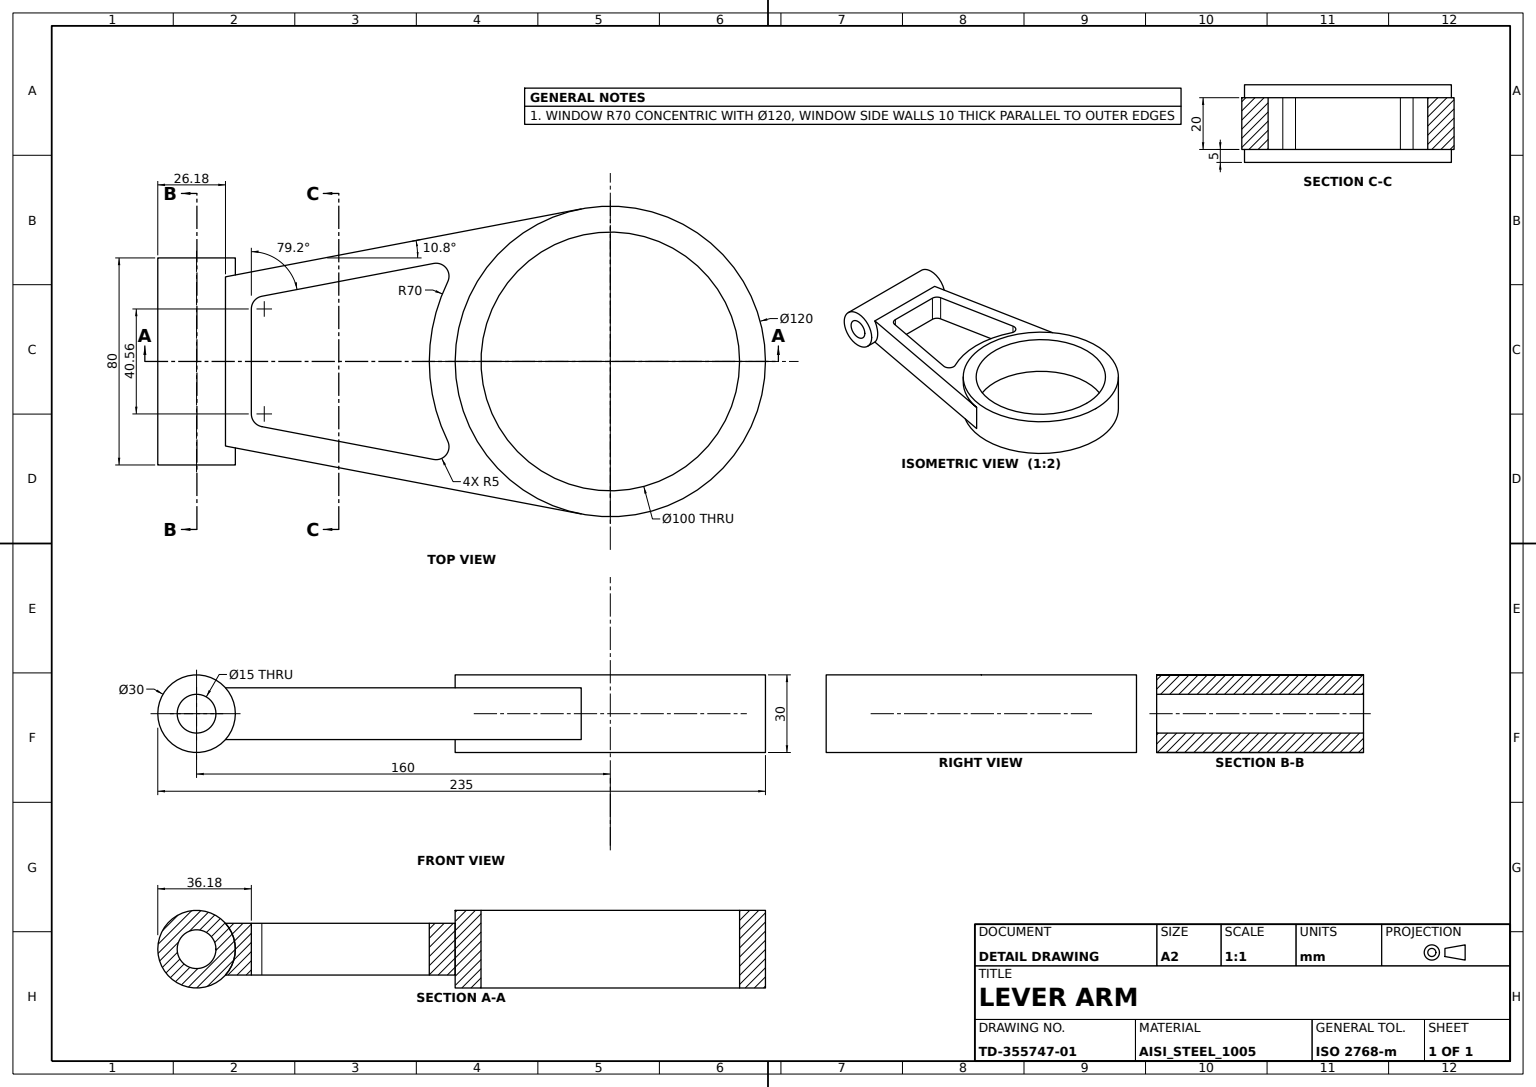
ISO-10303-21;
HEADER;
FILE_DESCRIPTION((''),'2;1');
FILE_NAME('','',(''),(''),'','','');
FILE_SCHEMA(('AUTOMOTIVE_DESIGN'));
ENDSEC;
DATA;
#1=APPLICATION_CONTEXT('');
#2=PRODUCT_CONTEXT('',#1,'mechanical');
#3=PRODUCT('','','',(#2));
#4=PRODUCT_DEFINITION_FORMATION('','',#3);
#5=PRODUCT_DEFINITION_CONTEXT('',#1,'design');
#6=PRODUCT_DEFINITION('','',#4,#5);
#7=PRODUCT_DEFINITION_SHAPE('','',#6);
#8=(LENGTH_UNIT()NAMED_UNIT(*)SI_UNIT(.MILLI.,.METRE.));
#9=(NAMED_UNIT(*)PLANE_ANGLE_UNIT()SI_UNIT($,.RADIAN.));
#10=(NAMED_UNIT(*)SI_UNIT($,.STERADIAN.)SOLID_ANGLE_UNIT());
#11=UNCERTAINTY_MEASURE_WITH_UNIT(LENGTH_MEASURE(0.005),#8,'distance_accuracy_value','');
#12=(GEOMETRIC_REPRESENTATION_CONTEXT(3)GLOBAL_UNCERTAINTY_ASSIGNED_CONTEXT((#11))GLOBAL_UNIT_ASSIGNED_CONTEXT((#8,#9,#10))REPRESENTATION_CONTEXT('',''));
#13=CARTESIAN_POINT('',(50.,0.,-15.));
#14=VERTEX_POINT('',#13);
#15=CARTESIAN_POINT('',(0.,0.,-15.));
#16=DIRECTION('',(0.,0.,-1.));
#17=DIRECTION('',(1.,0.,0.));
#18=AXIS2_PLACEMENT_3D('',#15,#16,#17);
#19=CIRCLE('',#18,50.);
#20=EDGE_CURVE('',#14,#14,#19,.T.);
#21=ORIENTED_EDGE('',*,*,#20,.T.);
#22=EDGE_LOOP('',(#21));
#23=FACE_BOUND('',#22,.T.);
#24=CARTESIAN_POINT('',(50.,0.,15.));
#25=VERTEX_POINT('',#24);
#26=CARTESIAN_POINT('',(0.,0.,15.));
#27=AXIS2_PLACEMENT_3D('',#26,#16,#17);
#28=CIRCLE('',#27,50.);
#29=EDGE_CURVE('',#25,#25,#28,.T.);
#30=ORIENTED_EDGE('',*,*,#29,.F.);
#31=EDGE_LOOP('',(#30));
#32=FACE_BOUND('',#31,.T.);
#33=DIRECTION('',(-1.,0.,0.));
#34=AXIS2_PLACEMENT_3D('',#26,#16,#33);
#35=CYLINDRICAL_SURFACE('',#34,50.);
#36=ADVANCED_FACE('',(#23,#32),#35,.F.);
#37=ORIENTED_EDGE('',*,*,#29,.T.);
#38=EDGE_LOOP('',(#37));
#39=FACE_BOUND('',#38,.T.);
#40=CARTESIAN_POINT('',(60.,0.,15.));
#41=VERTEX_POINT('',#40);
#42=CIRCLE('',#27,60.);
#43=EDGE_CURVE('',#41,#41,#42,.T.);
#44=ORIENTED_EDGE('',*,*,#43,.F.);
#45=EDGE_LOOP('',(#44));
#46=FACE_BOUND('',#45,.T.);
#47=PLANE('',#34);
#48=ADVANCED_FACE('',(#39,#46),#47,.F.);
#49=ORIENTED_EDGE('',*,*,#43,.T.);
#50=EDGE_LOOP('',(#49));
#51=FACE_BOUND('',#50,.T.);
#52=CARTESIAN_POINT('',(60.,0.,-15.));
#53=VERTEX_POINT('',#52);
#54=CIRCLE('',#18,60.);
#55=EDGE_CURVE('',#53,#53,#54,.T.);
#56=ORIENTED_EDGE('',*,*,#55,.F.);
#57=EDGE_LOOP('',(#56));
#58=FACE_BOUND('',#57,.T.);
#59=CYLINDRICAL_SURFACE('',#34,60.);
#60=ADVANCED_FACE('',(#51,#58),#59,.T.);
#61=ORIENTED_EDGE('',*,*,#20,.F.);
#62=EDGE_LOOP('',(#61));
#63=FACE_BOUND('',#62,.T.);
#64=ORIENTED_EDGE('',*,*,#55,.T.);
#65=EDGE_LOOP('',(#64));
#66=FACE_BOUND('',#65,.T.);
#67=AXIS2_PLACEMENT_3D('',#15,#16,#33);
#68=PLANE('',#67);
#69=ADVANCED_FACE('',(#63,#66),#68,.T.);
#70=CLOSED_SHELL('',(#36,#48,#60,#69));
#71=MANIFOLD_SOLID_BREP('',#70);
#72=CARTESIAN_POINT('',(-134.756787,25.189548,-10.));
#73=VERTEX_POINT('',#72);
#74=CARTESIAN_POINT('',(-138.81966,20.278154,-10.));
#75=VERTEX_POINT('',#74);
#76=CARTESIAN_POINT('',(-133.81966,20.278154,-10.));
#77=DIRECTION('',(0.,0.,1.));
#78=DIRECTION('',(0.982278847,0.187425366,0.));
#79=AXIS2_PLACEMENT_3D('',#76,#77,#78);
#80=CIRCLE('',#79,5.);
#81=EDGE_CURVE('',#73,#75,#80,.T.);
#82=ORIENTED_EDGE('',*,*,#81,.F.);
#83=CARTESIAN_POINT('',(-134.756787,25.189548,10.));
#84=VERTEX_POINT('',#83);
#85=VECTOR('',#77,1000.);
#86=LINE('',#72,#85);
#87=EDGE_CURVE('',#84,#73,#86,.F.);
#88=ORIENTED_EDGE('',*,*,#87,.F.);
#89=CARTESIAN_POINT('',(-138.81966,20.278154,10.));
#90=VERTEX_POINT('',#89);
#91=CARTESIAN_POINT('',(-133.81966,20.278154,10.));
#92=AXIS2_PLACEMENT_3D('',#91,#77,#78);
#93=CIRCLE('',#92,5.);
#94=EDGE_CURVE('',#84,#90,#93,.T.);
#95=ORIENTED_EDGE('',*,*,#94,.T.);
#96=LINE('',#74,#85);
#97=EDGE_CURVE('',#90,#75,#96,.F.);
#98=ORIENTED_EDGE('',*,*,#97,.T.);
#99=EDGE_LOOP('',(#82,#88,#95,#98));
#100=FACE_BOUND('',#99,.T.);
#101=AXIS2_PLACEMENT_3D('',#76,#77,#17);
#102=CYLINDRICAL_SURFACE('',#101,5.);
#103=ADVANCED_FACE('',(#100),#102,.F.);
#104=CARTESIAN_POINT('',(-62.879481,-30.759891,10.));
#105=VERTEX_POINT('',#104);
#106=CARTESIAN_POINT('',(-62.879481,30.759891,10.));
#107=VERTEX_POINT('',#106);
#108=CARTESIAN_POINT('',(0.,0.,10.));
#109=AXIS2_PLACEMENT_3D('',#108,#16,#78);
#110=CIRCLE('',#109,70.);
#111=EDGE_CURVE('',#105,#107,#110,.T.);
#112=ORIENTED_EDGE('',*,*,#111,.T.);
#113=CARTESIAN_POINT('',(-62.879481,30.759891,-10.));
#114=VERTEX_POINT('',#113);
#115=LINE('',#113,#85);
#116=EDGE_CURVE('',#107,#114,#115,.F.);
#117=ORIENTED_EDGE('',*,*,#116,.T.);
#118=CARTESIAN_POINT('',(-62.879481,-30.759891,-10.));
#119=VERTEX_POINT('',#118);
#120=CARTESIAN_POINT('',(0.,0.,-10.));
#121=AXIS2_PLACEMENT_3D('',#120,#16,#78);
#122=CIRCLE('',#121,70.);
#123=EDGE_CURVE('',#119,#114,#122,.T.);
#124=ORIENTED_EDGE('',*,*,#123,.F.);
#125=LINE('',#118,#85);
#126=EDGE_CURVE('',#105,#119,#125,.F.);
#127=ORIENTED_EDGE('',*,*,#126,.F.);
#128=EDGE_LOOP('',(#112,#117,#124,#127));
#129=FACE_BOUND('',#128,.T.);
#130=AXIS2_PLACEMENT_3D('',#120,#77,#17);
#131=CYLINDRICAL_SURFACE('',#130,70.);
#132=ADVANCED_FACE('',(#129),#131,.T.);
#133=CARTESIAN_POINT('',(-68.307999,-37.86842,10.));
#134=VERTEX_POINT('',#133);
#135=CARTESIAN_POINT('',(-67.370872,-32.957026,10.));
#136=AXIS2_PLACEMENT_3D('',#135,#77,#78);
#137=CIRCLE('',#136,5.);
#138=EDGE_CURVE('',#134,#105,#137,.T.);
#139=ORIENTED_EDGE('',*,*,#138,.F.);
#140=CARTESIAN_POINT('',(-134.756787,-25.189548,10.));
#141=VERTEX_POINT('',#140);
#142=DIRECTION('',(0.982278847,-0.187425366,0.));
#143=VECTOR('',#142,1000.);
#144=LINE('',#140,#143);
#145=EDGE_CURVE('',#141,#134,#144,.T.);
#146=ORIENTED_EDGE('',*,*,#145,.F.);
#147=CARTESIAN_POINT('',(-138.81966,-20.278154,10.));
#148=VERTEX_POINT('',#147);
#149=CARTESIAN_POINT('',(-133.81966,-20.278154,10.));
#150=AXIS2_PLACEMENT_3D('',#149,#77,#78);
#151=CIRCLE('',#150,5.);
#152=EDGE_CURVE('',#148,#141,#151,.T.);
#153=ORIENTED_EDGE('',*,*,#152,.F.);
#154=DIRECTION('',(0.,-1.,0.));
#155=VECTOR('',#154,1000.);
#156=LINE('',#89,#155);
#157=EDGE_CURVE('',#90,#148,#156,.T.);
#158=ORIENTED_EDGE('',*,*,#157,.F.);
#159=ORIENTED_EDGE('',*,*,#94,.F.);
#160=CARTESIAN_POINT('',(-68.307999,37.86842,10.));
#161=VERTEX_POINT('',#160);
#162=DIRECTION('',(-0.982278847,-0.187425366,0.));
#163=VECTOR('',#162,1000.);
#164=LINE('',#160,#163);
#165=EDGE_CURVE('',#161,#84,#164,.T.);
#166=ORIENTED_EDGE('',*,*,#165,.F.);
#167=CARTESIAN_POINT('',(-67.370872,32.957026,10.));
#168=AXIS2_PLACEMENT_3D('',#167,#77,#78);
#169=CIRCLE('',#168,5.);
#170=EDGE_CURVE('',#107,#161,#169,.T.);
#171=ORIENTED_EDGE('',*,*,#170,.F.);
#172=ORIENTED_EDGE('',*,*,#111,.F.);
#173=EDGE_LOOP('',(#139,#146,#153,#158,#159,#166,#171,#172));
#174=FACE_BOUND('',#173,.T.);
#175=CARTESIAN_POINT('',(-11.245522,-58.936731,10.));
#176=VERTEX_POINT('',#175);
#177=CARTESIAN_POINT('',(-148.81966,-32.686666,10.));
#178=VERTEX_POINT('',#177);
#179=CARTESIAN_POINT('',(-136.427008,-35.051267,10.));
#180=DIRECTION('',(-0.982278847,0.187425366,0.));
#181=VECTOR('',#180,1000.);
#182=LINE('',#179,#181);
#183=EDGE_CURVE('',#176,#178,#182,.T.);
#184=ORIENTED_EDGE('',*,*,#183,.F.);
#185=CARTESIAN_POINT('',(-11.245522,58.936731,10.));
#186=VERTEX_POINT('',#185);
#187=AXIS2_PLACEMENT_3D('',#108,#77,#17);
#188=CIRCLE('',#187,60.);
#189=EDGE_CURVE('',#186,#176,#188,.T.);
#190=ORIENTED_EDGE('',*,*,#189,.F.);
#191=CARTESIAN_POINT('',(-148.81966,32.686666,10.));
#192=VERTEX_POINT('',#191);
#193=CARTESIAN_POINT('',(-173.247802,28.025613,10.));
#194=VECTOR('',#78,1000.);
#195=LINE('',#193,#194);
#196=EDGE_CURVE('',#192,#186,#195,.T.);
#197=ORIENTED_EDGE('',*,*,#196,.F.);
#198=CARTESIAN_POINT('',(-148.81966,-100.,10.));
#199=DIRECTION('',(0.,1.,0.));
#200=VECTOR('',#199,1000.);
#201=LINE('',#198,#200);
#202=EDGE_CURVE('',#178,#192,#201,.T.);
#203=ORIENTED_EDGE('',*,*,#202,.F.);
#204=EDGE_LOOP('',(#184,#190,#197,#203));
#205=FACE_BOUND('',#204,.T.);
#206=AXIS2_PLACEMENT_3D('',#198,#77,#17);
#207=PLANE('',#206);
#208=ADVANCED_FACE('',(#174,#205),#207,.T.);
#209=CARTESIAN_POINT('',(-148.81966,32.686666,-10.));
#210=VERTEX_POINT('',#209);
#211=CARTESIAN_POINT('',(-160.,30.553383,0.));
#212=DIRECTION('',(0.187425366,-0.982278847,0.));
#213=AXIS2_PLACEMENT_3D('',#211,#212,#78);
#214=ELLIPSE('',#213,15.270613,15.);
#215=EDGE_CURVE('',#210,#192,#214,.T.);
#216=ORIENTED_EDGE('',*,*,#215,.F.);
#217=CARTESIAN_POINT('',(-148.81966,-32.686666,-10.));
#218=VERTEX_POINT('',#217);
#219=CARTESIAN_POINT('',(-148.81966,-100.,-10.));
#220=LINE('',#219,#200);
#221=EDGE_CURVE('',#218,#210,#220,.T.);
#222=ORIENTED_EDGE('',*,*,#221,.F.);
#223=CARTESIAN_POINT('',(-160.,-30.553383,0.));
#224=DIRECTION('',(0.187425366,0.982278847,0.));
#225=AXIS2_PLACEMENT_3D('',#223,#224,#180);
#226=ELLIPSE('',#225,15.270613,15.);
#227=EDGE_CURVE('',#178,#218,#226,.T.);
#228=ORIENTED_EDGE('',*,*,#227,.F.);
#229=ORIENTED_EDGE('',*,*,#202,.T.);
#230=EDGE_LOOP('',(#216,#222,#228,#229));
#231=FACE_BOUND('',#230,.T.);
#232=CARTESIAN_POINT('',(-160.,-100.,0.));
#233=AXIS2_PLACEMENT_3D('',#232,#199,#77);
#234=CYLINDRICAL_SURFACE('',#233,15.);
#235=ADVANCED_FACE('',(#231),#234,.F.);
#236=CARTESIAN_POINT('',(-138.81966,-20.278154,-10.));
#237=VERTEX_POINT('',#236);
#238=LINE('',#74,#155);
#239=EDGE_CURVE('',#75,#237,#238,.T.);
#240=ORIENTED_EDGE('',*,*,#239,.F.);
#241=ORIENTED_EDGE('',*,*,#97,.F.);
#242=ORIENTED_EDGE('',*,*,#157,.T.);
#243=LINE('',#236,#85);
#244=EDGE_CURVE('',#148,#237,#243,.F.);
#245=ORIENTED_EDGE('',*,*,#244,.T.);
#246=EDGE_LOOP('',(#240,#241,#242,#245));
#247=FACE_BOUND('',#246,.T.);
#248=AXIS2_PLACEMENT_3D('',#74,#33,#77);
#249=PLANE('',#248);
#250=ADVANCED_FACE('',(#247),#249,.F.);
#251=ORIENTED_EDGE('',*,*,#165,.T.);
#252=ORIENTED_EDGE('',*,*,#87,.T.);
#253=CARTESIAN_POINT('',(-68.307999,37.86842,-10.));
#254=VERTEX_POINT('',#253);
#255=LINE('',#253,#163);
#256=EDGE_CURVE('',#254,#73,#255,.T.);
#257=ORIENTED_EDGE('',*,*,#256,.F.);
#258=LINE('',#253,#85);
#259=EDGE_CURVE('',#161,#254,#258,.F.);
#260=ORIENTED_EDGE('',*,*,#259,.F.);
#261=EDGE_LOOP('',(#251,#252,#257,#260));
#262=FACE_BOUND('',#261,.T.);
#263=DIRECTION('',(-0.187425366,0.982278847,0.));
#264=AXIS2_PLACEMENT_3D('',#253,#263,#162);
#265=PLANE('',#264);
#266=ADVANCED_FACE('',(#262),#265,.F.);
#267=CARTESIAN_POINT('',(-11.245522,58.936731,-10.));
#268=VERTEX_POINT('',#267);
#269=CARTESIAN_POINT('',(-11.245522,58.936731,40.));
#270=VECTOR('',#16,1000.);
#271=LINE('',#269,#270);
#272=EDGE_CURVE('',#186,#268,#271,.T.);
#273=ORIENTED_EDGE('',*,*,#272,.F.);
#274=ORIENTED_EDGE('',*,*,#189,.T.);
#275=CARTESIAN_POINT('',(-11.245522,-58.936731,-10.));
#276=VERTEX_POINT('',#275);
#277=CARTESIAN_POINT('',(-11.245522,-58.936731,40.));
#278=LINE('',#277,#270);
#279=EDGE_CURVE('',#176,#276,#278,.T.);
#280=ORIENTED_EDGE('',*,*,#279,.T.);
#281=AXIS2_PLACEMENT_3D('',#120,#16,#33);
#282=CIRCLE('',#281,60.);
#283=EDGE_CURVE('',#276,#268,#282,.T.);
#284=ORIENTED_EDGE('',*,*,#283,.T.);
#285=EDGE_LOOP('',(#273,#274,#280,#284));
#286=FACE_BOUND('',#285,.T.);
#287=CARTESIAN_POINT('',(0.,0.,40.));
#288=AXIS2_PLACEMENT_3D('',#287,#16,#33);
#289=CYLINDRICAL_SURFACE('',#288,60.);
#290=ADVANCED_FACE('',(#286),#289,.F.);
#291=CARTESIAN_POINT('',(-68.307999,-37.86842,-10.));
#292=VERTEX_POINT('',#291);
#293=LINE('',#291,#85);
#294=EDGE_CURVE('',#134,#292,#293,.F.);
#295=ORIENTED_EDGE('',*,*,#294,.T.);
#296=CARTESIAN_POINT('',(-134.756787,-25.189548,-10.));
#297=VERTEX_POINT('',#296);
#298=LINE('',#296,#143);
#299=EDGE_CURVE('',#297,#292,#298,.T.);
#300=ORIENTED_EDGE('',*,*,#299,.F.);
#301=LINE('',#296,#85);
#302=EDGE_CURVE('',#141,#297,#301,.F.);
#303=ORIENTED_EDGE('',*,*,#302,.F.);
#304=ORIENTED_EDGE('',*,*,#145,.T.);
#305=EDGE_LOOP('',(#295,#300,#303,#304));
#306=FACE_BOUND('',#305,.T.);
#307=DIRECTION('',(-0.187425366,-0.982278847,0.));
#308=AXIS2_PLACEMENT_3D('',#296,#307,#142);
#309=PLANE('',#308);
#310=ADVANCED_FACE('',(#306),#309,.F.);
#311=CARTESIAN_POINT('',(-133.81966,-20.278154,-10.));
#312=AXIS2_PLACEMENT_3D('',#311,#77,#78);
#313=CIRCLE('',#312,5.);
#314=EDGE_CURVE('',#237,#297,#313,.T.);
#315=ORIENTED_EDGE('',*,*,#314,.F.);
#316=ORIENTED_EDGE('',*,*,#244,.F.);
#317=ORIENTED_EDGE('',*,*,#152,.T.);
#318=ORIENTED_EDGE('',*,*,#302,.T.);
#319=EDGE_LOOP('',(#315,#316,#317,#318));
#320=FACE_BOUND('',#319,.T.);
#321=AXIS2_PLACEMENT_3D('',#311,#77,#17);
#322=CYLINDRICAL_SURFACE('',#321,5.);
#323=ADVANCED_FACE('',(#320),#322,.F.);
#324=ORIENTED_EDGE('',*,*,#279,.F.);
#325=ORIENTED_EDGE('',*,*,#183,.T.);
#326=ORIENTED_EDGE('',*,*,#227,.T.);
#327=CARTESIAN_POINT('',(-3.685611,-60.379212,-10.));
#328=LINE('',#327,#143);
#329=EDGE_CURVE('',#218,#276,#328,.T.);
#330=ORIENTED_EDGE('',*,*,#329,.T.);
#331=EDGE_LOOP('',(#324,#325,#326,#330));
#332=FACE_BOUND('',#331,.T.);
#333=CARTESIAN_POINT('',(-162.900227,-30.,40.));
#334=AXIS2_PLACEMENT_3D('',#333,#224,#180);
#335=PLANE('',#334);
#336=ADVANCED_FACE('',(#332),#335,.F.);
#337=ORIENTED_EDGE('',*,*,#215,.T.);
#338=ORIENTED_EDGE('',*,*,#196,.T.);
#339=ORIENTED_EDGE('',*,*,#272,.T.);
#340=CARTESIAN_POINT('',(-40.506405,53.353559,-10.));
#341=LINE('',#340,#163);
#342=EDGE_CURVE('',#268,#210,#341,.T.);
#343=ORIENTED_EDGE('',*,*,#342,.T.);
#344=EDGE_LOOP('',(#337,#338,#339,#343));
#345=FACE_BOUND('',#344,.T.);
#346=AXIS2_PLACEMENT_3D('',#269,#212,#78);
#347=PLANE('',#346);
#348=ADVANCED_FACE('',(#345),#347,.F.);
#349=ORIENTED_EDGE('',*,*,#342,.F.);
#350=ORIENTED_EDGE('',*,*,#283,.F.);
#351=ORIENTED_EDGE('',*,*,#329,.F.);
#352=ORIENTED_EDGE('',*,*,#221,.T.);
#353=EDGE_LOOP('',(#349,#350,#351,#352));
#354=FACE_BOUND('',#353,.T.);
#355=ORIENTED_EDGE('',*,*,#81,.T.);
#356=ORIENTED_EDGE('',*,*,#239,.T.);
#357=ORIENTED_EDGE('',*,*,#314,.T.);
#358=ORIENTED_EDGE('',*,*,#299,.T.);
#359=CARTESIAN_POINT('',(-67.370872,-32.957026,-10.));
#360=AXIS2_PLACEMENT_3D('',#359,#77,#78);
#361=CIRCLE('',#360,5.);
#362=EDGE_CURVE('',#292,#119,#361,.T.);
#363=ORIENTED_EDGE('',*,*,#362,.T.);
#364=ORIENTED_EDGE('',*,*,#123,.T.);
#365=CARTESIAN_POINT('',(-67.370872,32.957026,-10.));
#366=AXIS2_PLACEMENT_3D('',#365,#77,#78);
#367=CIRCLE('',#366,5.);
#368=EDGE_CURVE('',#114,#254,#367,.T.);
#369=ORIENTED_EDGE('',*,*,#368,.T.);
#370=ORIENTED_EDGE('',*,*,#256,.T.);
#371=EDGE_LOOP('',(#355,#356,#357,#358,#363,#364,#369,#370));
#372=FACE_BOUND('',#371,.T.);
#373=CARTESIAN_POINT('',(-11.245522,-100.,-10.));
#374=AXIS2_PLACEMENT_3D('',#373,#16,#33);
#375=PLANE('',#374);
#376=ADVANCED_FACE('',(#354,#372),#375,.T.);
#377=ORIENTED_EDGE('',*,*,#126,.T.);
#378=ORIENTED_EDGE('',*,*,#362,.F.);
#379=ORIENTED_EDGE('',*,*,#294,.F.);
#380=ORIENTED_EDGE('',*,*,#138,.T.);
#381=EDGE_LOOP('',(#377,#378,#379,#380));
#382=FACE_BOUND('',#381,.T.);
#383=AXIS2_PLACEMENT_3D('',#359,#77,#17);
#384=CYLINDRICAL_SURFACE('',#383,5.);
#385=ADVANCED_FACE('',(#382),#384,.F.);
#386=ORIENTED_EDGE('',*,*,#259,.T.);
#387=ORIENTED_EDGE('',*,*,#368,.F.);
#388=ORIENTED_EDGE('',*,*,#116,.F.);
#389=ORIENTED_EDGE('',*,*,#170,.T.);
#390=EDGE_LOOP('',(#386,#387,#388,#389));
#391=FACE_BOUND('',#390,.T.);
#392=AXIS2_PLACEMENT_3D('',#365,#77,#17);
#393=CYLINDRICAL_SURFACE('',#392,5.);
#394=ADVANCED_FACE('',(#391),#393,.F.);
#395=CLOSED_SHELL('',(#103,#132,#208,#235,#250,#266,#290,#310,#323,#336,#348,#376,#385,#394));
#396=MANIFOLD_SOLID_BREP('',#395);
#397=CARTESIAN_POINT('',(-145.,-40.,0.));
#398=VERTEX_POINT('',#397);
#399=CARTESIAN_POINT('',(-160.,-40.,0.));
#400=AXIS2_PLACEMENT_3D('',#399,#154,#17);
#401=CIRCLE('',#400,15.);
#402=EDGE_CURVE('',#398,#398,#401,.T.);
#403=ORIENTED_EDGE('',*,*,#402,.F.);
#404=EDGE_LOOP('',(#403));
#405=FACE_BOUND('',#404,.T.);
#406=CARTESIAN_POINT('',(-145.,40.,0.));
#407=VERTEX_POINT('',#406);
#408=CARTESIAN_POINT('',(-160.,40.,0.));
#409=AXIS2_PLACEMENT_3D('',#408,#154,#17);
#410=CIRCLE('',#409,15.);
#411=EDGE_CURVE('',#407,#407,#410,.T.);
#412=ORIENTED_EDGE('',*,*,#411,.T.);
#413=EDGE_LOOP('',(#412));
#414=FACE_BOUND('',#413,.T.);
#415=AXIS2_PLACEMENT_3D('',#399,#199,#77);
#416=CYLINDRICAL_SURFACE('',#415,15.);
#417=ADVANCED_FACE('',(#405,#414),#416,.T.);
#418=CARTESIAN_POINT('',(-152.5,-40.,0.));
#419=VERTEX_POINT('',#418);
#420=CIRCLE('',#400,7.5);
#421=EDGE_CURVE('',#419,#419,#420,.T.);
#422=ORIENTED_EDGE('',*,*,#421,.T.);
#423=EDGE_LOOP('',(#422));
#424=FACE_BOUND('',#423,.T.);
#425=CARTESIAN_POINT('',(-152.5,40.,0.));
#426=VERTEX_POINT('',#425);
#427=CIRCLE('',#409,7.5);
#428=EDGE_CURVE('',#426,#426,#427,.T.);
#429=ORIENTED_EDGE('',*,*,#428,.F.);
#430=EDGE_LOOP('',(#429));
#431=FACE_BOUND('',#430,.T.);
#432=CYLINDRICAL_SURFACE('',#415,7.5);
#433=ADVANCED_FACE('',(#424,#431),#432,.F.);
#434=ORIENTED_EDGE('',*,*,#402,.T.);
#435=EDGE_LOOP('',(#434));
#436=FACE_BOUND('',#435,.T.);
#437=ORIENTED_EDGE('',*,*,#421,.F.);
#438=EDGE_LOOP('',(#437));
#439=FACE_BOUND('',#438,.T.);
#440=AXIS2_PLACEMENT_3D('',#399,#154,#16);
#441=PLANE('',#440);
#442=ADVANCED_FACE('',(#436,#439),#441,.T.);
#443=ORIENTED_EDGE('',*,*,#411,.F.);
#444=EDGE_LOOP('',(#443));
#445=FACE_BOUND('',#444,.T.);
#446=ORIENTED_EDGE('',*,*,#428,.T.);
#447=EDGE_LOOP('',(#446));
#448=FACE_BOUND('',#447,.T.);
#449=AXIS2_PLACEMENT_3D('',#408,#154,#16);
#450=PLANE('',#449);
#451=ADVANCED_FACE('',(#445,#448),#450,.F.);
#452=CLOSED_SHELL('',(#417,#433,#442,#451));
#453=MANIFOLD_SOLID_BREP('',#452);
#454=ADVANCED_BREP_SHAPE_REPRESENTATION('',(#71,#396,#453),#12);
#455=SHAPE_DEFINITION_REPRESENTATION(#7,#454);
ENDSEC;
END-ISO-10303-21;
